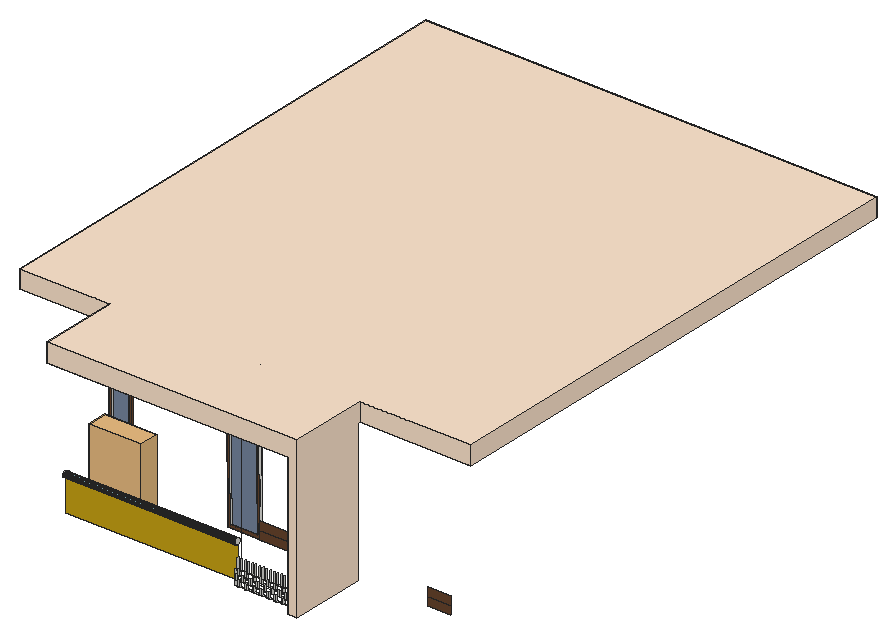
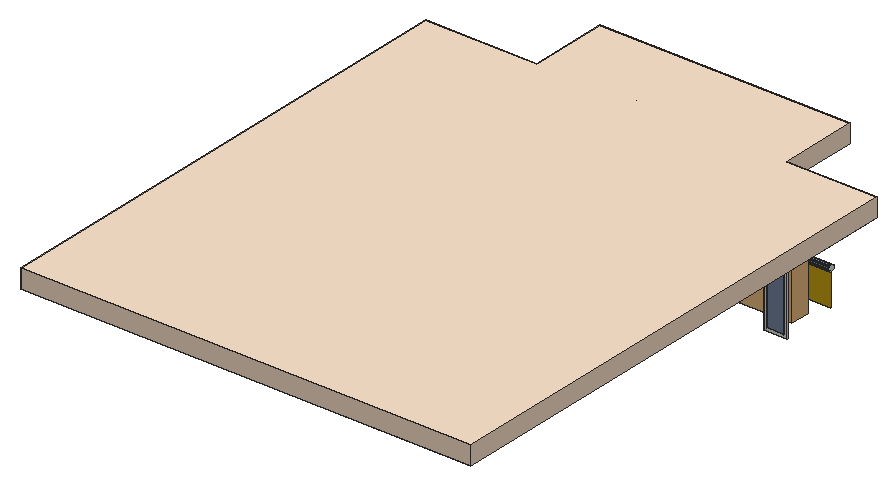
# SketchUp Ruby script. Lengths in inches.
U = 1.inch
M = Sketchup.active_model
def pt(a) = Geom::Point3d.new(a.map { |v| v * U })
def face(e, loops, mat)
  f = e.add_face(loops[0].map { |a| pt(a) })
  loops[1..].each { |l| e.add_face(l.map { |a| pt(a) }).erase! }
  f.material = f.back_material = mat if mat
  f
end
# faces: each face lists its corners as indices into pts; further lists are holes
def faces(e, pts, list, mat = nil) = list.each { |f| face(e, (f[0].is_a?(Array) ? f : [f]).map { |l| l.map { |i| pts[i] } }, mat) }
# xy, xz, yz: faces in a plane at the given z, y or x. An outline is a flat list of corners, or four numbers for a rectangle; further outlines are holes
def ring(l) = l.size == 4 ? [[l[0], l[1]], [l[2], l[1]], [l[2], l[3]], [l[0], l[3]]] : l.each_slice(2).to_a
def flat(e, list, mat, &to3) = list.each { |f| face(e, (f[0].is_a?(Array) ? f : [f]).map { |l| ring(l).map { |u, v| to3.(u, v) } }, mat) }
def xy(e, z, list, mat = nil) = flat(e, list, mat) { |x, y| [x, y, z] }
def xz(e, y, list, mat = nil) = flat(e, list, mat) { |x, z| [x, y, z] }
def yz(e, x, list, mat = nil) = flat(e, list, mat) { |y, z| [x, y, z] }
def lines(e, pts, list) = list.each { |a, b| e.add_line(pt(pts[a]), pt(pts[b])) }
# prism: a flat outline (further loops are holes) pulled along v
def prism(e, loops, v, mat = nil)
  f = face(e, loops, mat); d = Geom::Vector3d.new(v.map { |x| x * U })
  f.pushpull(f.normal.samedirection?(d) ? d.length : -d.length)
end
def box(e, o, s, mat = nil) = prism(e, [[o, [o[0] + s[0], o[1], o[2]], [o[0] + s[0], o[1] + s[1], o[2]], [o[0], o[1] + s[1], o[2]]]], [0, 0, s[2]], mat)
def at(x, y, z, deg = 0) = Geom::Transformation.translation(pt([x, y, z])) * Geom::Transformation.rotation(ORIGIN, Z_AXIS, deg.degrees)
def axes(o, x, y, z) = Geom::Transformation.new([*x, 0, *y, 0, *z, 0, *pt(o).to_a, 1])
def part(name) = M.definitions.add(name)
# library, detail: a bought-in or finely detailed component or shape, given as its bounding box
def library(name, o, s) = part(name).tap { |d| box(d.entities, o, s) }
def detail(e, o, s) = box(e.add_group.entities, o, s)
def put(e, d, t, mat = nil) = e.add_instance(d, t).tap { |i| i.material = mat if mat }
def group(e, t, mat = nil) = e.add_group.tap { |g| g.transformation = t; g.material = mat if mat }.entities
root = M.entities
M.materials.add("C01_Vanilla_Cream").color = [255, 230, 206]
M.materials.add("Glass_Mirror_01").color = [119, 135, 160]
M.materials.add("Metal_Cladding_01_1K").color = [126, 169, 182]
M.materials.add("Metal_Perforated_08_1K").color = [201, 163, 22]
M.materials.add("Wood_Veneer_15_1K").color = [103, 69, 45]
c1 = library("Group_2",[-1.28,-0.39,0],[21.22,20.51,48.44])
xy(root,297.09,[[283.14,137.21,284.89,138.74],[290.55,137.21,292.3,138.74],[297.96,137.21,299.71,138.74],[305.37,137.21,307.12,138.74],[312.78,137.21,314.53,138.74],
  [320.1875,137.21,321.94,138.74],[327.6,137.21,329.35,138.74],[335.01,137.21,336.76,138.74],[342.42,137.21,344.17,138.74]])
xy(root,297.49,[[280.31,137.21,282.27,138.74],[285.76,137.21,289.68,138.74],[293.17,137.21,297.09,138.74],[300.58,137.21,304.5,138.74],[307.99,137.21,311.91,138.74],
  [315.4,137.21,319.32,138.74],[322.81,137.21,326.73,138.74],[330.22,137.21,334.14,138.74],[337.63,137.21,341.55,138.74],[345.04,137.21,347,138.74]])
xy(root,301.97,[[100.9,200,124.11,201]])
xy(root,302.36,[[281.18,137.21,283.14,138.74],[284.89,137.21,286.85,138.74],[288.59,137.21,290.55,138.74],[292.3,137.21,294.26,138.74],[296,137.21,297.96,138.74],
  [299.71,137.21,301.67,138.74],[303.41,137.21,305.37,138.74],[307.12,137.21,309.08,138.74],[310.82,137.21,312.78,138.74],[314.53,137.21,316.49,138.74],
  [318.23,137.21,320.1875,138.74],[321.94,137.21,323.9,138.74],[325.64,137.21,327.6,138.74],[329.35,137.21,331.31,138.74],[333.05,137.21,335.01,138.74],
  [336.76,137.21,338.72,138.74],[340.46,137.21,342.42,138.74],[344.17,137.21,346.13,138.74]])
xy(root,304.97,[[103.9,200,121.11,201]])
xy(root,307.72,[[281.18,137.21,283.14,138.74],[284.89,137.21,286.85,138.74],[288.59,137.21,290.55,138.74],[292.3,137.21,294.26,138.74],[296,137.21,297.96,138.74],
  [299.71,137.21,301.67,138.74],[303.41,137.21,305.37,138.74],[307.12,137.21,309.08,138.74],[310.82,137.21,312.78,138.74],[314.53,137.21,316.49,138.74],
  [318.23,137.21,320.1875,138.74],[321.94,137.21,323.9,138.74],[325.64,137.21,327.6,138.74],[329.35,137.21,331.31,138.74],[333.05,137.21,335.01,138.74],
  [336.76,137.21,338.72,138.74],[340.46,137.21,342.42,138.74],[344.17,137.21,346.13,138.74]])
xy(root,312.59,[[280.31,137.21,282.27,138.74],[285.76,137.21,289.68,138.74],[293.17,137.21,297.09,138.74],[300.58,137.21,304.5,138.74],[307.99,137.21,311.91,138.74],
  [315.4,137.21,319.32,138.74],[322.81,137.21,326.73,138.74],[330.22,137.21,334.14,138.74],[337.63,137.21,341.55,138.74],[345.04,137.21,347,138.74]])
xy(root,312.99,[[283.14,137.21,284.89,138.74],[290.55,137.21,292.3,138.74],[297.96,137.21,299.71,138.74],[305.37,137.21,307.12,138.74],[312.78,137.21,314.53,138.74],
  [320.1875,137.21,321.94,138.74],[327.6,137.21,329.35,138.74],[335.01,137.21,336.76,138.74],[342.42,137.21,344.17,138.74]])
xy(root,419,[[103.9,200,121.11,201]])
xy(root,422,[[100.9,200,124.11,201]])
xz(root,138.6875,[[105.48,302,282.125,335.2]],"Metal_Perforated_08_1K")
xz(root,198,[[256.9,303.92,357,312.6],[429,303.92,453,312.6],[256.9,312.6,357,321.28],[429,312.6,453,321.28]],"Wood_Veneer_15_1K")
xz(root,200,[[[100.9,301.97,124.11,422],[103.9,304.97,121.11,419]]],"Wood_Veneer_15_1K")
xz(root,201,[[[100.9,301.97,124.11,422],[103.9,304.97,121.11,419]],[256.33,302,256.9,422]])
xz(root,201,[[103.9,304.97,121.11,419]],"Glass_Mirror_01")
yz(root,100.9,[[200,301.97,201,422]])
yz(root,103.9,[[200,304.97,201,419]])
yz(root,105.48,[[137.9375,335.1,137.1875,335.2,136.49,335.49,135.89,335.95,135.42,336.55,135.13,337.25,135.04,338,135.13,338.75,135.42,339.45,135.89,340.05,136.49,340.51,137.1875,340.8,137.9375,340.9,138.6875,340.8,139.39,340.51,139.99,340.05,140.45,339.45,140.74,338.75,140.84,338,140.74,337.25,140.45,336.55,139.99,335.95,139.39,335.49,138.6875,335.2]])
yz(root,121.11,[[200,304.97,201,419]],"Wood_Veneer_15_1K")
yz(root,124.11,[[200,301.97,201,422]],"Wood_Veneer_15_1K")
yz(root,220.99,[[201.92,301.98,199.92,422.92,201,422.93,203,302]])
yz(root,223.99,[[201.87,304.98,202.95,305,201.05,419.93,199.97,419.92]])
yz(root,251.32,[[201.87,304.98,199.97,419.92,201.05,419.93,202.95,305]])
yz(root,254.32,[[201.92,301.98,203,302,201,422.9,201,422.93,199.92,422.92]])
yz(root,280.31,[[137.21,297.49,138.74,312.59]])
yz(root,281.18,[[137.21,302.36,138.74,307.72]])
yz(root,282.125,[[137.9375,335.1,138.6875,335.2,139.39,335.49,139.99,335.95,140.45,336.55,140.74,337.25,140.84,338,140.74,338.75,140.45,339.45,139.99,340.05,139.39,340.51,138.6875,340.8,137.9375,340.9,137.21,340.8,137.1875,340.8,136.49,340.51,135.89,340.05,135.42,339.45,135.13,338.75,135.04,338,135.13,337.25,135.42,336.55,135.89,335.95,136.49,335.49,137.1875,335.2,137.21,335.2]])
yz(root,282.27,[[137.21,312.59,138.74,323.12]])
yz(root,283.14,[[137.21,297.09,138.74,302.36],[137.21,307.72,138.74,312.99]])
yz(root,284.89,[[137.21,297.09,138.74,302.36],[137.21,307.72,138.74,312.99]])
yz(root,285.76,[[137.21,312.59,138.74,323.12]])
yz(root,286.85,[[137.21,302.36,138.74,307.72]])
yz(root,288.59,[[137.21,302.36,138.74,307.72]])
yz(root,289.68,[[137.21,312.59,138.74,323.12]])
yz(root,290.55,[[137.21,297.09,138.74,302.36],[137.21,307.72,138.74,312.99]])
yz(root,292.3,[[137.21,297.09,138.74,302.36],[137.21,307.72,138.74,312.99]])
yz(root,293.17,[[137.21,312.59,138.74,323.12]])
yz(root,294.26,[[137.21,302.36,138.74,307.72]])
yz(root,296,[[137.21,302.36,138.74,307.72]])
yz(root,297.09,[[137.21,312.59,138.74,323.12]])
yz(root,297.96,[[137.21,297.09,138.74,302.36],[137.21,307.72,138.74,312.99]])
yz(root,299.71,[[137.21,297.09,138.74,302.36],[137.21,307.72,138.74,312.99]])
yz(root,300.58,[[137.21,312.59,138.74,323.12]])
yz(root,301.67,[[137.21,302.36,138.74,307.72]])
yz(root,303.41,[[137.21,302.36,138.74,307.72]])
yz(root,304.5,[[137.21,312.59,138.74,323.12]])
yz(root,305.37,[[137.21,297.09,138.74,302.36],[137.21,307.72,138.74,312.99]])
yz(root,307.12,[[137.21,297.09,138.74,302.36],[137.21,307.72,138.74,312.99]])
yz(root,307.99,[[137.21,312.59,138.74,323.12]])
yz(root,309.08,[[137.21,302.36,138.74,307.72]])
yz(root,310.82,[[137.21,302.36,138.74,307.72]])
yz(root,311.91,[[137.21,312.59,138.74,323.12]])
yz(root,312.78,[[137.21,297.09,138.74,302.36],[137.21,307.72,138.74,312.99]])
yz(root,314.53,[[137.21,297.09,138.74,302.36],[137.21,307.72,138.74,312.99]])
yz(root,315.4,[[137.21,312.59,138.74,323.12]])
yz(root,316.49,[[137.21,302.36,138.74,307.72]])
yz(root,318.23,[[137.21,302.36,138.74,307.72]])
yz(root,319.32,[[137.21,312.59,138.74,323.12]])
yz(root,320.1875,[[137.21,297.09,138.74,302.36],[137.21,307.72,138.74,312.99]])
yz(root,321.94,[[137.21,297.09,138.74,302.36],[137.21,307.72,138.74,312.99]])
yz(root,322.81,[[137.21,312.59,138.74,323.12]])
yz(root,323.9,[[137.21,302.36,138.74,307.72]])
yz(root,325.64,[[137.21,302.36,138.74,307.72]])
yz(root,326.73,[[137.21,312.59,138.74,323.12]])
yz(root,327.6,[[137.21,297.09,138.74,302.36],[137.21,307.72,138.74,312.99]])
yz(root,329.35,[[137.21,297.09,138.74,302.36],[137.21,307.72,138.74,312.99]])
yz(root,330.22,[[137.21,312.59,138.74,323.12]])
yz(root,331.31,[[137.21,302.36,138.74,307.72]])
yz(root,333.05,[[137.21,302.36,138.74,307.72]])
yz(root,334.14,[[137.21,312.59,138.74,323.12]])
yz(root,335.01,[[137.21,297.09,138.74,302.36],[137.21,307.72,138.74,312.99]])
yz(root,336.76,[[137.21,297.09,138.74,302.36],[137.21,307.72,138.74,312.99]])
yz(root,337.63,[[137.21,312.59,138.74,323.12]])
yz(root,338.72,[[137.21,302.36,138.74,307.72]])
yz(root,340.46,[[137.21,302.36,138.74,307.72]])
yz(root,341.55,[[137.21,312.59,138.74,323.12]])
yz(root,342.42,[[137.21,297.09,138.74,302.36],[137.21,307.72,138.74,312.99]])
yz(root,344.17,[[137.21,297.09,138.74,302.36],[137.21,307.72,138.74,312.99]])
yz(root,345.04,[[137.21,312.59,138.74,323.12]])
yz(root,346.13,[[137.21,302.36,138.74,307.72]])
yz(root,347,[[137.21,297.49,138.74,312.59]])
p = [[254.32,199.92,422.92],[220.99,199.92,422.92],[220.99,201.92,301.98],[254.32,201.92,301.98],[223.99,201.87,304.98],[223.99,199.97,419.92],
  [251.32,199.97,419.92],[251.32,201.87,304.98],[256.33,199.92,422.92],[254.32,201,302],[256.33,201,302],[220.99,201,422.93],
  [254.32,201,422.93],[254.32,201,422.9],[254.32,203,302],[220.99,203,302],[223.99,201.05,419.93],[223.99,202.95,305],
  [251.32,202.95,305],[251.32,201.05,419.93],[105.48,137.1875,335.2],[105.48,137.9375,335.1],[282.125,137.9375,335.1],[282.125,137.21,335.2],
  [282.125,137.1875,335.2],[105.48,138.6875,335.2],[282.125,138.6875,335.2],[105.48,136.49,335.49],[282.125,136.49,335.49],[105.48,139.39,335.49],
  [282.125,139.39,335.49],[105.48,135.89,335.95],[282.125,135.89,335.95],[105.48,139.99,335.95],[282.125,139.99,335.95],[105.48,135.42,336.55],
  [282.125,135.42,336.55],[105.48,140.45,336.55],[282.125,140.45,336.55],[105.48,135.13,337.25],[282.125,135.13,337.25],[105.48,140.74,337.25],
  [282.125,140.74,337.25],[105.48,135.04,338],[282.125,135.04,338],[105.48,140.84,338],[282.125,140.84,338],[105.48,135.13,338.75],
  [282.125,135.13,338.75],[105.48,140.74,338.75],[282.125,140.74,338.75],[105.48,135.42,339.45],[282.125,135.42,339.45],[105.48,140.45,339.45],
  [282.125,140.45,339.45],[105.48,135.89,340.05],[282.125,135.89,340.05],[105.48,139.99,340.05],[282.125,139.99,340.05],[105.48,136.49,340.51],
  [282.125,136.49,340.51],[105.48,139.39,340.51],[282.125,139.39,340.51],[105.48,137.1875,340.8],[282.125,137.1875,340.8],[105.48,138.6875,340.8],
  [282.125,138.6875,340.8],[105.48,137.9375,340.9],[282.125,137.21,340.8],[282.125,137.9375,340.9],[347,120.55,302],[347,142.6875,302],
  [347,142.6875,446],[282.16,143.21,302],[282.16,143.21,446],[346.97,136.6875,302],[282.125,137.21,302]]
faces(root,p,[[[0,1,2,3],[4,5,6,7]]],"Wood_Veneer_15_1K")
faces(root,p,[[8,0,9,10],[[11,12,13,14,15],[16,17,18,19]],[15,14,3,2],[18,17,4,7]])
faces(root,p,[[16,17,18,19]],"Glass_Mirror_01")
faces(root,p,[[20,21,22,23,24],[21,25,26,22],[27,20,24,28],[25,29,30,26],[31,27,28,32],[29,33,34,30],[35,31,32,36],[33,37,38,34],
  [39,35,36,40],[37,41,42,38],[43,39,40,44],[41,45,46,42],[47,43,44,48],[45,49,50,46],[51,47,48,52],[49,53,54,50],
  [55,51,52,56],[53,57,58,54],[59,55,56,60],[57,61,62,58],[63,59,60,64],[61,65,66,62],[67,63,64,68,69],[65,67,69,66]],"Metal_Cladding_01_1K")
lines(root,p,[[70,71],[72,71],[71,73],[73,74],[71,75],[73,76]])
put(root,c1,axes([117.26,158.08,302],[2.485,0,0],[0,1,0],[0,0,1.57]))
g1 = group(root,at(9,201,446),"C01_Vanilla_Cream")
xy(g1,-144,[[338,-80.45,348,-3]])
xy(g1,0,[[91.9,-80.45,91.9,0,0,0,0,519,462,519,462,0,348,0,348,-3,338,-3,338,-80.45]])
xy(g1,19,[[91.9,-80.45,348,-80.45,348,0,462,0,462,519,0,519,0,0,91.9,0]])
xz(g1,-80.45,[[338,-144,348,-144,348,19,91.9,19,91.9,0,338,0]])
xz(g1,-3,[[338,-144,348,0]])
xz(g1,0,[[0,0,91.9,19],[348,0,462,19]])
xz(g1,519,[[0,0,462,19]])
yz(g1,0,[[0,0,519,19]])
yz(g1,91.9,[[-80.45,0,0,19]])
yz(g1,338,[[-80.45,-144,-3,0]])
yz(g1,348,[[-80.45,-144,-3,-144,-3,0,0,0,0,19,-80.45,19]])
yz(g1,462,[[0,0,519,19]])
p = [[247.9,0,0],[247.9,0,-0.11],[247.9,-3,19],[247.9,-3,1.14]]
lines(g1,p,[[0,1],[2,3]])
